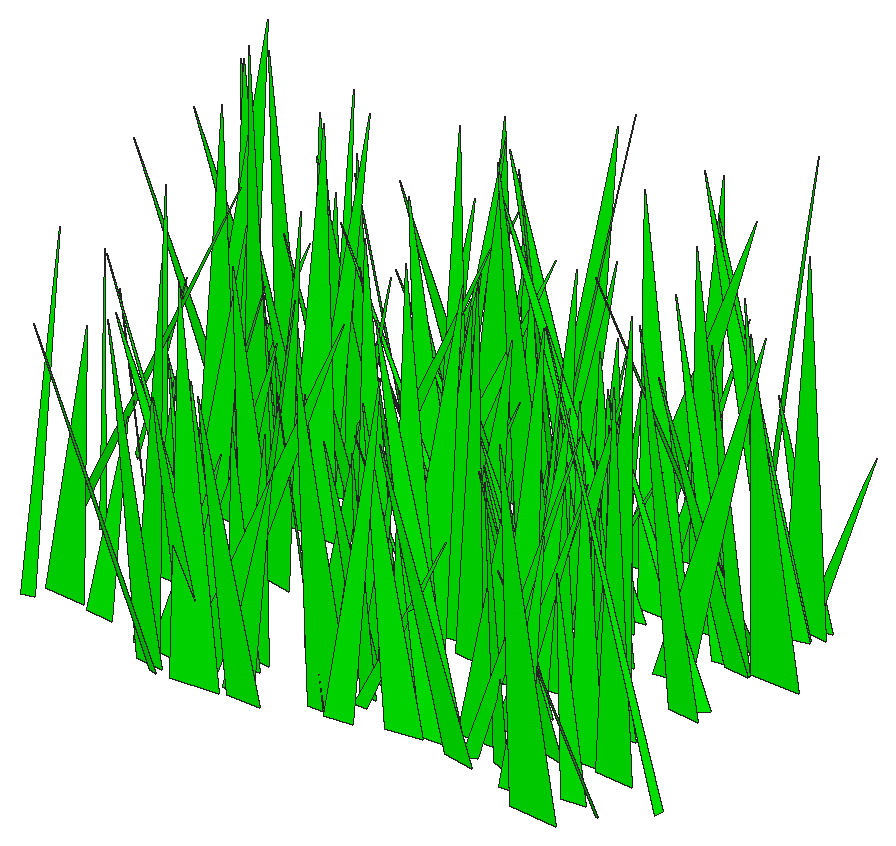
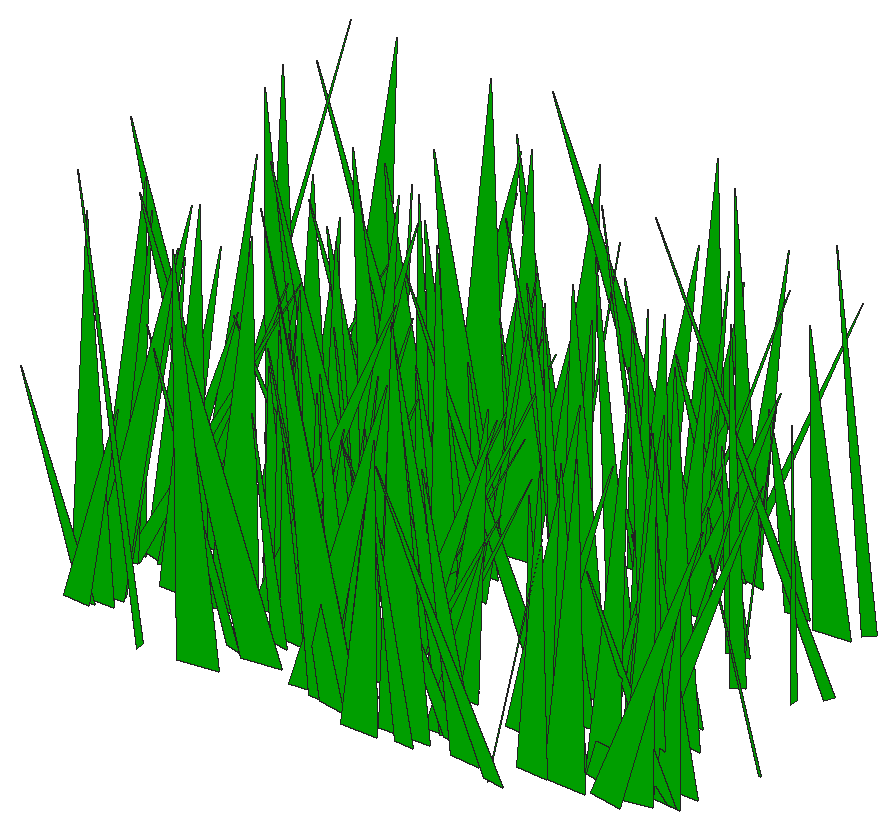
# SketchUp Ruby script. Lengths in inches.
U = 1.inch
M = Sketchup.active_model
def pt(a) = Geom::Point3d.new(a.map { |v| v * U })
def face(e, loops, mat)
  f = e.add_face(loops[0].map { |a| pt(a) })
  loops[1..].each { |l| e.add_face(l.map { |a| pt(a) }).erase! }
  f.material = f.back_material = mat if mat
  f
end
# faces: each face lists its corners as indices into pts; further lists are holes
def faces(e, pts, list, mat = nil) = list.each { |f| face(e, (f[0].is_a?(Array) ? f : [f]).map { |l| l.map { |i| pts[i] } }, mat) }
# xy, xz, yz: faces in a plane at the given z, y or x. An outline is a flat list of corners, or four numbers for a rectangle; further outlines are holes
def ring(l) = l.size == 4 ? [[l[0], l[1]], [l[2], l[1]], [l[2], l[3]], [l[0], l[3]]] : l.each_slice(2).to_a
def flat(e, list, mat, &to3) = list.each { |f| face(e, (f[0].is_a?(Array) ? f : [f]).map { |l| ring(l).map { |u, v| to3.(u, v) } }, mat) }
def xy(e, z, list, mat = nil) = flat(e, list, mat) { |x, y| [x, y, z] }
def xz(e, y, list, mat = nil) = flat(e, list, mat) { |x, z| [x, y, z] }
def yz(e, x, list, mat = nil) = flat(e, list, mat) { |y, z| [x, y, z] }
def lines(e, pts, list) = list.each { |a, b| e.add_line(pt(pts[a]), pt(pts[b])) }
# prism: a flat outline (further loops are holes) pulled along v
def prism(e, loops, v, mat = nil)
  f = face(e, loops, mat); d = Geom::Vector3d.new(v.map { |x| x * U })
  f.pushpull(f.normal.samedirection?(d) ? d.length : -d.length)
end
def box(e, o, s, mat = nil) = prism(e, [[o, [o[0] + s[0], o[1], o[2]], [o[0] + s[0], o[1] + s[1], o[2]], [o[0], o[1] + s[1], o[2]]]], [0, 0, s[2]], mat)
def at(x, y, z, deg = 0) = Geom::Transformation.translation(pt([x, y, z])) * Geom::Transformation.rotation(ORIGIN, Z_AXIS, deg.degrees)
def axes(o, x, y, z) = Geom::Transformation.new([*x, 0, *y, 0, *z, 0, *pt(o).to_a, 1])
def part(name) = M.definitions.add(name)
# library, detail: a bought-in or finely detailed component or shape, given as its bounding box
def library(name, o, s) = part(name).tap { |d| box(d.entities, o, s) }
def detail(e, o, s) = box(e.add_group.entities, o, s)
def put(e, d, t, mat = nil) = e.add_instance(d, t).tap { |i| i.material = mat if mat }
def group(e, t, mat = nil) = e.add_group.tap { |g| g.transformation = t; g.material = mat if mat }.entities
root = M.entities
M.materials.add("[0065_Lime]").color = [0, 255, 0]
c1 = part("fur_instance\#9")
p = [[0.8125,0,1.79],[0.67,-0.02,1.48],[0,-0.11,0],[0,0.11,0]]
faces(c1.entities,p,[[0,1,2,3]])
put(root,c1,axes([86.03,28.1875,1.48],[4.04083,0.10334,0.71067],[-0.84468,0.57426,0.37961],[-0.76857,-0.0878,3.31922]),"[0065_Lime]")
put(root,c1,axes([88.59,32.07,1.48],[-3.94525,-0.72329,0.33492],[5.16377,-0.55267,0.25148],[0.00431,0.07235,5.26929]),"[0065_Lime]")
put(root,c1,axes([87.08,31.14,1.48],[0.89992,-0.6126,0.18107],[4.3401,0.12899,0.35137],[-0.46837,0.0182,3.60385]),"[0065_Lime]")
put(root,c1,axes([87.77,31.65,1.48],[-5.27126,0.64585,1.86007],[-4.76084,-0.78731,0.23364],[1.92071,-0.17899,5.68396]),"[0065_Lime]")
put(root,c1,axes([89.39,29.05,1.48],[-5.37329,-0.53147,0.49477],[3.82303,-0.75334,0.35434],[0.24449,0.09936,5.33315]),"[0065_Lime]")
put(root,c1,axes([88.04,30.97,1.48],[0.57285,1.047,1.52629],[-7.66011,0.0985,-0.36204],[-0.60113,-0.25748,6.06786]),"[0065_Lime]")
put(root,c1,axes([87.96,24.23,1.48],[-5.20678,0.05391,1.90036],[-0.24332,-0.80109,0.32044],[2.35503,0.03643,4.23464]),"[0065_Lime]")
put(root,c1,axes([87.5,30.42,1.48],[1.19423,1.25105,0.91528],[-8.97397,0.16665,0.11422],[-0.00931,-0.15934,7.30591]),"[0065_Lime]")
put(root,c1,axes([87.07,31.14,1.48],[3.31324,0.45192,0.12553],[-3.21982,0.46497,0.13723],[0.00691,-0.03211,3.7534]),"[0065_Lime]")
put(root,c1,axes([89.58,31.27,1.48],[-2.8313,-0.4498,0.75727],[3.31009,-0.39968,0.23348],[0.39536,0.12512,3.46825]),"[0065_Lime]")
put(root,c1,axes([89.35,31.25,1.48],[4.48601,0.7755,2.98863],[-6.12778,0.72297,-0.20054],[-2.53145,-0.37579,5.78163]),"[0065_Lime]")
put(root,c1,axes([89.05,28.11,1.48],[-2.78497,-0.8522,3.3684],[7.24104,-0.42235,0.38055],[1.2235,0.55979,5.41505]),"[0065_Lime]")
put(root,c1,axes([88.17,28.92,1.48],[4.25422,-0.04589,0.62894],[0.27567,0.60656,0.24919],[-0.79279,-0.03533,3.46166]),"[0065_Lime]")
put(root,c1,axes([88.69,19.89,1.48],[7.16155,-0.18947,2.24815],[1.59238,1.07053,-0.33303],[-2.63082,0.13221,5.91829]),"[0065_Lime]")
put(root,c1,axes([89.9,28.91,1.48],[-6.41024,-0.72474,2.92404],[5.66582,-0.9786,0.09049],[2.7244,0.32992,6.69179]),"[0065_Lime]")
put(root,c1,axes([90.01,32.15,1.48],[1.06489,-0.86721,2.0596],[6.63418,0.17535,0.20448],[-0.69739,0.34385,5.09006]),"[0065_Lime]")
put(root,c1,axes([89.72,24.6,1.48],[-6.42583,0.25596,2.56922],[-1.98471,-0.99997,0.05395],[3.05869,-0.11112,5.43254]),"[0065_Lime]")
put(root,c1,axes([90.54,23.32,1.48],[-5.24025,-0.12439,1.38818],[0.80005,-0.77419,-0.32639],[1.74817,-0.01856,4.31054]),"[0065_Lime]")
put(root,c1,axes([89.62,27.03,1.48],[2.51456,0.77635,0.8023],[-5.5838,0.36135,-0.13764],[-0.56446,-0.11612,4.93568]),"[0065_Lime]")
put(root,c1,axes([89.54,20.53,1.48],[0.63715,-0.86567,0.6252],[6.19645,0.08196,-0.37544],[0.38378,0.11385,5.0238]),"[0065_Lime]")
put(root,c1,axes([91.32,25.14,1.48],[-4.16997,0.13533,0.69258],[-1.02836,-0.59488,-0.20161],[0.77135,-0.06148,3.47535]),"[0065_Lime]")
put(root,c1,axes([87.27,23.48,1.48],[9.017,-0.09495,0.44591],[0.68586,1.26911,-0.12098],[-0.53545,0.02663,7.35411]),"[0065_Lime]")
put(root,c1,axes([91.93,33.24,1.48],[-5.20309,-0.09303,1.05154],[0.59415,-0.75284,-0.28659],[1.32532,-0.02771,4.25674]),"[0065_Lime]")
put(root,c1,axes([90.71,31.09,1.48],[2.09408,-0.8014,0.72809],[5.74409,0.30262,0.23064],[-0.57723,0.10406,4.93651]),"[0065_Lime]")
put(root,c1,axes([91.21,32.15,1.48],[-3.10372,-0.68812,1.8346],[5.2342,-0.47225,-0.07664],[1.29263,0.26005,4.71534]),"[0065_Lime]")
put(root,c1,axes([90.89,23.12,1.48],[-1.58701,0.49138,1.36255],[-3.73837,-0.26141,0.27803],[1.02908,-0.19183,3.11127]),"[0065_Lime]")
put(root,c1,axes([91.02,20.25,1.48],[0.34432,0.60128,0.49992],[-4.31408,0.04225,0.2632],[0.27666,-0.08952,3.48194]),"[0065_Lime]")
put(root,c1,axes([90.48,26.84,1.48],[2.13067,-0.53653,0.37097],[3.84241,0.29416,-0.34537],[0.1516,0.08493,3.53984]),"[0065_Lime]")
put(root,c1,axes([92.04,26.2,1.48],[0.50197,-0.76027,1.37562],[5.63187,0.09401,0.38125],[-0.64443,0.22937,4.40337]),"[0065_Lime]")
put(root,c1,axes([93.5625,22.1,1.48],[-4.52451,0.50099,0.28299],[-3.58217,-0.63323,-0.32904],[0.02176,-0.07491,4.67404]),"[0065_Lime]")
put(root,c1,axes([92.68,30.49,1.48],[-0.96712,-1.02503,0.3105],[7.29873,-0.13343,0.28177],[-0.29375,0.05952,5.97885]),"[0065_Lime]")
put(root,c1,axes([94.25,18.65,1.48],[-6.30246,-0.24518,0.48424],[1.78851,-0.88542,0.37897],[0.44746,0.08562,5.30583]),"[0065_Lime]")
put(root,c1,axes([93.55,28.98,1.48],[-4.67422,-0.41949,0.77765],[3.07015,-0.66133,0.25562],[0.63279,0.10996,4.50412]),"[0065_Lime]")
put(root,c1,axes([91.95,29.78,1.48],[7.64496,-0.26622,2.61897],[2.13429,1.15701,-0.18107],[-3.0661,0.14159,6.40407]),"[0065_Lime]")
put(root,c1,axes([94.74,21.09,1.48],[-7.30199,0.04274,0.76879],[-0.26383,-1.0338,0.26771],[0.95717,0.04107,5.93865]),"[0065_Lime]")
put(root,c1,axes([92.59,30.31,1.48],[-2.98365,-0.45574,1.59582],[3.49222,-0.46692,-0.14825],[1.47394,0.18373,3.58161]),"[0065_Lime]")
put(root,c1,axes([91.89,29.12,1.48],[7.25302,-0.57073,1.92647],[4.19021,1.06216,0.10651],[-2.1327,0.14589,6.76094]),"[0065_Lime]")
put(root,c1,axes([92.83,27.71,1.48],[-2.87939,1.03833,2.40511],[-7.82216,-0.45076,0.32479],[1.46925,-0.3649,6.4426]),"[0065_Lime]")
put(root,c1,axes([93.88,18.95,1.48],[-4.81384,-0.61573,1.676],[4.63408,-0.70422,0.13728],[1.40405,0.21323,5.29314]),"[0065_Lime]")
put(root,c1,axes([93.29,19.57,1.48],[5.72947,0.66066,2.42178],[-5.06339,0.86801,-0.00891],[-2.30906,-0.26411,6.0287]),"[0065_Lime]")
put(root,c1,axes([94.0625,21.62,1.48],[-2.35642,0.53998,1.63788],[-4.29031,-0.33785,-0.35163],[0.64414,-0.27487,3.64976]),"[0065_Lime]")
put(root,c1,axes([94.35,21.02,1.48],[-2.68065,0.46037,0.38934],[-3.27201,-0.38158,0.21344],[0.5069,-0.02846,3.4367]),"[0065_Lime]")
put(root,c1,axes([91.73,33.25,1.48],[4.99894,0.51633,0.09697],[-3.67616,0.70236,0.07104],[-0.04431,-0.01981,5.04603]),"[0065_Lime]")
put(root,c1,axes([94.77,31.97,1.48],[-2.33051,0.57135,0.33218],[-4.08624,-0.32507,-0.23277],[-0.04652,-0.06976,3.80501]),"[0065_Lime]")
put(root,c1,axes([93.15,32.78,1.48],[2.93751,0.70108,0.9852],[-5.09923,0.42123,0.01537],[-0.59788,-0.14804,4.70946]),"[0065_Lime]")
put(root,c1,axes([93.83,24.81,1.48],[-5.24364,-0.63249,2.99099],[5.05891,-0.83929,-0.07906],[2.86155,0.32477,5.62059]),"[0065_Lime]")
put(root,c1,axes([95.17,19.42,1.48],[-5.76861,0.18281,1.60389],[-1.23906,-0.85663,0.32311],[2.01126,-0.00342,4.79925]),"[0065_Lime]")
put(root,c1,axes([93.83,19.65,1.48],[2.04566,0.60081,0.00556],[-4.27557,0.28744,0.02824],[0.02837,-0.00297,3.85534]),"[0065_Lime]")
put(root,c1,axes([95.64,29.99,1.48],[-1.88741,0.91938,0.41555],[-6.56263,-0.26403,-0.14749],[-0.03316,-0.07603,5.53705]),"[0065_Lime]")
put(root,c1,axes([95.7,18.93,1.48],[-2.98711,-0.68925,0.80252],[4.96925,-0.42751,-0.06573],[0.58313,0.1124,4.67103]),"[0065_Lime]")
put(root,c1,axes([96.9,31.13,1.48],[-4.86899,0.11572,0.16903],[-0.83851,-0.68199,-0.33524],[0.13538,-0.06201,4.00274]),"[0065_Lime]")
put(root,c1,axes([96.79,31.51,1.48],[-4.52046,-0.72566,0.40008],[5.18576,-0.63453,0.20271],[0.13575,0.07509,5.57892]),"[0065_Lime]")
put(root,c1,axes([94.98,31.66,1.48],[3.7016,0.2066,1.14464],[-1.42051,0.55619,-0.3245],[-1.45743,-0.01737,3.22346]),"[0065_Lime]")
put(root,c1,axes([95.69,18.76,1.48],[1.77449,-0.98089,3.05276],[7.83983,0.29649,0.17716],[-1.16223,0.50238,5.856]),"[0065_Lime]")
put(root,c1,axes([94.32,31.9,1.48],[6.98938,-0.44614,1.69614],[3.31092,1.01631,-0.06941],[-1.86182,0.13249,6.24395]),"[0065_Lime]")
put(root,c1,axes([97.31,28.75,1.48],[-4.58533,-0.17957,0.22713],[1.28519,-0.64509,0.07713],[0.24342,0.02339,3.87113]),"[0065_Lime]")
put(root,c1,axes([95.11,33.125,1.48],[3.44674,0.43758,1.26928],[-3.35812,0.49936,0.26484],[-0.92475,-0.18245,3.76911]),"[0065_Lime]")
put(root,c1,axes([95.38,32.76,1.48],[0.6225,-1.16517,1.07209],[8.3925,0.08091,-0.27771],[0.24611,0.18817,6.75811]),"[0065_Lime]")
put(root,c1,axes([94.14,32.09,1.48],[4.70239,0.5043,0.09383],[-3.59067,0.66055,0.09974],[-0.01727,-0.02353,4.81066]),"[0065_Lime]")
put(root,c1,axes([96.13,20.46,1.48],[0.86751,-0.7228,0.53652],[5.16693,0.12851,0.27388],[-0.44412,0.08327,4.23433]),"[0065_Lime]")
put(root,c1,axes([95.29,21.59,1.48],[-6.1048,-0.27843,3.1373],[2.11287,-1.0083,-0.27832],[3.78658,0.11373,5.21332]),"[0065_Lime]")
put(root,c1,axes([96.64,33.28,1.48],[-1.92502,0.75297,1.78022],[-5.76376,-0.27916,-0.16715],[0.53227,-0.2997,4.62844]),"[0065_Lime]")
put(root,c1,axes([96.07,21.03,1.48],[-0.49663,-0.67233,0.88373],[4.87395,-0.08523,-0.3605],[0.56361,0.14461,3.89615]),"[0065_Lime]")
put(root,c1,axes([99.14,27.45,1.48],[-7.16847,0.07697,0.30495],[-0.54164,-1.00857,0.10615],[0.3837,0.0143,5.84696]),"[0065_Lime]")
put(root,c1,axes([93.95,28.14,1.48],[7.45779,-0.35097,0.2333],[2.48234,1.04795,0.32467],[-0.39846,-0.04044,6.38919]),"[0065_Lime]")
put(root,c1,axes([97.35,18.92,1.48],[-2.46713,-0.78531,0.91792],[5.69029,-0.34997,0.0861],[0.3572,0.15115,4.96842]),"[0065_Lime]")
put(root,c1,axes([96.51,29.41,1.48],[6.69522,-0.63939,2.8413],[4.98924,1.02135,-0.07697],[-2.83087,0.28786,6.58422]),"[0065_Lime]")
put(root,c1,axes([95.8,29.52,1.48],[4.45032,-0.60961,0.8059],[4.36425,0.63637,0.18455],[-0.86934,0.074,5.05199]),"[0065_Lime]")
put(root,c1,axes([97.29,22.42,1.48],[-2.1606,-0.65244,1.23513],[4.81878,-0.32297,-0.13947],[0.8024,0.18274,4.16334]),"[0065_Lime]")
put(root,c1,axes([98.05,32.4375,1.48],[-6.44509,-0.25277,1.83432],[1.95631,-0.95304,0.14724],[2.11994,0.11101,5.44089]),"[0065_Lime]")
put(root,c1,axes([97.23,28.5625,1.48],[3.46289,0.39438,1.48863],[-3.01998,0.52757,-0.03533],[-1.45127,-0.15679,3.62557]),"[0065_Lime]")
put(root,c1,axes([99.34,27.22,1.48],[-4.93591,-0.10561,0.07686],[0.75703,-0.69088,0.35484],[0.02738,0.0626,4.04568]),"[0065_Lime]")
put(root,c1,axes([96.52,23.78,1.48],[6.35659,0.55025,1.45954],[-3.94858,0.92398,-0.29436],[-1.72114,-0.08756,6.06575]),"[0065_Lime]")
put(root,c1,axes([99.25,32.31,1.48],[-4.77874,0.84226,0.2925],[-5.99757,-0.67265,0.0721],[0.29354,-0.03173,6.23502]),"[0065_Lime]")
put(root,c1,axes([98.61,25.18,1.48],[-6.59327,-0.28209,1.56863],[1.99347,-0.96474,-0.26958],[1.94294,0.03258,5.59965]),"[0065_Lime]")
put(root,c1,axes([96.93,19.1875,1.48],[1.56737,-0.67288,0.6223],[4.84771,0.2145,-0.30665],[0.12507,0.11855,4.08696]),"[0065_Lime]")
put(root,c1,axes([95.14,19.74,1.48],[7.49911,-0.68292,0.41068],[4.87795,1.05389,-0.20878],[-0.2837,0.06888,7.26587]),"[0065_Lime]")
put(root,c1,axes([98.33,30.73,1.48],[-0.36242,0.81621,0.08718],[-5.80927,-0.05076,-0.05253],[-0.05779,-0.01559,4.73366]),"[0065_Lime]")
put(root,c1,axes([98.79,27.62,1.48],[-3.13529,-0.49774,1.52243],[3.83228,-0.46996,0.07325],[1.16778,0.20592,3.8471]),"[0065_Lime]")
put(root,c1,axes([99.44,19.91,1.48],[-5.81231,-0.14491,1.45485],[1.20351,-0.8479,0.35128],[1.67752,0.10622,4.78878]),"[0065_Lime]")
put(root,c1,axes([98.07,32.6,1.48],[2.15064,1.21441,0.14312],[-8.6398,0.3028,-0.19535],[-0.27558,-0.01583,7.2416]),"[0065_Lime]")
put(root,c1,axes([99.375,22.21,1.48],[-2.55361,-0.60704,0.26531],[4.31243,-0.36126,-0.23464],[0.41455,0.01872,4.07521]),"[0065_Lime]")
put(root,c1,axes([98.09,32.7,1.48],[3.66492,0.61612,0.90487],[-4.46208,0.52544,-0.03086],[-0.74307,-0.11645,4.64821]),"[0065_Lime]")
put(root,c1,axes([99.3125,22.64,1.48],[-4.21624,1.01487,2.01393],[-7.48842,-0.62718,0.21788],[1.48885,-0.28051,6.79908]),"[0065_Lime]")
put(root,c1,axes([97.49,27.8,1.48],[4.4356,-0.266,0.15227],[1.88004,0.62319,0.24381],[-0.28958,-0.02846,3.91522]),"[0065_Lime]")
put(root,c1,axes([98.73,31.34,1.48],[4.06229,-0.59453,1.3386],[4.35948,0.59745,0.13825],[-1.2666,0.14956,4.76902]),"[0065_Lime]")
put(root,c1,axes([99.77,19.88,1.48],[-0.48716,-1.05909,0.61167],[7.57237,-0.06561,0.18373],[-0.17803,0.10746,6.14078]),"[0065_Lime]")
put(root,c1,axes([99.07,22.46,1.48],[3.60187,0.40609,1.09838],[-2.98977,0.52954,-0.07358],[-1.112,-0.10839,3.75557]),"[0065_Lime]")
put(root,c1,axes([97.88,31.875,1.48],[9.08789,0.18976,1.8378],[-1.3943,1.31498,0.01214],[-2.23256,-0.0488,7.47337]),"[0065_Lime]")
put(root,c1,axes([99.96,21.33,1.48],[-3.57418,-0.39045,1.45708],[3.0397,-0.53388,0.13951],[1.3,0.17484,3.67986]),"[0065_Lime]")
put(root,c1,axes([99.39,23.96,1.48],[2.52048,-0.47153,0.541],[3.36444,0.36269,0.22159],[-0.61914,0.05129,3.40654]),"[0065_Lime]")
put(root,c1,axes([100.52,28.47,1.48],[-4.96564,-1.01095,1.93745],[7.41374,-0.73099,-0.20922],[1.57182,0.25406,7.10758]),"[0065_Lime]")
put(root,c1,axes([101.8,22.69,1.48],[-4.96831,0.00753,0.31786],[-0.07995,-0.69866,-0.2724],[0.38624,-0.04779,4.03233]),"[0065_Lime]")
put(root,c1,axes([99.48,25.42,1.48],[3.80749,-0.88549,1.00747],[6.35385,0.54883,0.27603],[-0.93437,0.1238,5.98245]),"[0065_Lime]")
put(root,c1,axes([99.4,26.99,1.48],[1.5064,-0.91139,0.26779],[6.4863,0.20879,-0.33085],[0.32234,0.05792,5.40607]),"[0065_Lime]")
put(root,c1,axes([103.09,29.5,1.48],[-7.20756,0.53099,0.20381],[-3.76765,-1.01304,0.283],[0.38334,0.02699,6.61356]),"[0065_Lime]")
put(root,c1,axes([101.37,29.86,1.48],[-4.19113,0.24642,0.83769],[-1.75907,-0.60561,0.14656],[1.0206,-0.03187,3.69261]),"[0065_Lime]")
put(root,c1,axes([100.18,19.74,1.48],[-5.21221,0.52408,3.00978],[-4.14292,-0.8604,0.27331],[3.23078,-0.25781,5.20614]),"[0065_Lime]")
put(root,c1,axes([100.86,24.87,1.48],[5.2899,0.68458,2.31174],[-5.15837,0.80864,-0.21424],[-2.28098,-0.24109,5.84573]),"[0065_Lime]")
put(root,c1,axes([100.49,22.94,1.48],[0.74059,1.18616,0.87624],[-8.50522,0.09817,0.30313],[0.28017,-0.15526,6.88603]),"[0065_Lime]")
put(root,c1,axes([102.14,20.27,1.48],[-2.00366,0.86038,0.7845],[-6.197,-0.275,-0.36601],[-0.1332,-0.14837,5.22757]),"[0065_Lime]")
put(root,c1,axes([101.32,30.49,1.48],[0.96996,0.53402,0.84598],[-3.9249,0.14416,-0.07176],[-0.34557,-0.1384,3.18954]),"[0065_Lime]")
put(root,c1,axes([103.04,26.02,1.48],[-3.3694,0.40735,0.10034],[-2.8989,-0.47147,-0.27056],[-0.12377,-0.04672,3.60535]),"[0065_Lime]")
put(root,c1,axes([101.13,27.57,1.48],[5.20611,-0.04577,1.54913],[0.49937,0.77488,-0.3432],[-1.86649,0.07965,4.22909]),"[0065_Lime]")
put(root,c1,axes([102.22,20.83,1.48],[-2.02806,1.27509,1.24963],[-9.19603,-0.28959,0.02683],[0.36771,-0.20965,7.56316]),"[0065_Lime]")
put(root,c1,axes([100.14,20.78,1.48],[4.05172,-0.24086,0.16976],[1.72615,0.56698,-0.3023],[-0.04656,0.05954,3.56573]),"[0065_Lime]")
put(root,c1,axes([100.8125,29.6,1.48],[5.18578,0.26596,1.00114],[-1.8663,0.7488,-0.2696],[-1.27054,-0.01437,4.48226]),"[0065_Lime]")
put(root,c1,axes([101.75,28.8,1.48],[3.18601,-0.39642,1.19727],[2.86771,0.48455,0.32695],[-1.37901,0.09176,3.44603]),"[0065_Lime]")
put(root,c1,axes([103.38,20.52,1.48],[-4.95266,0.95785,0.21261],[-6.80269,-0.69687,0.35626],[0.50794,0.00652,6.84444]),"[0065_Lime]")
put(root,c1,axes([101.48,30.84,1.48],[3.52892,0.37904,1.08038],[-2.80358,0.5188,-0.0402],[-1.08648,-0.10758,3.6128]),"[0065_Lime]")
put(root,c1,axes([102.6,28.85,1.48],[-2.41907,0.6927,0.73234],[-4.94324,-0.35291,0.3821],[0.82251,-0.08369,4.45025]),"[0065_Lime]")
put(root,c1,axes([102.21,29.37,1.48],[1.06039,-0.73807,1.72179],[5.65967,0.14852,-0.1728],[-0.19466,0.29768,4.35525]),"[0065_Lime]")
put(root,c1,axes([103.68,30.2,1.48],[-2.9082,1.16047,0.54886],[-8.26636,-0.41325,0.2984],[0.57097,-0.07218,7.11569]),"[0065_Lime]")
put(root,c1,axes([104.33,20.02,1.48],[-4.09177,-0.69665,0.43226],[4.96433,-0.57822,-0.13422],[0.46585,0.04276,5.22706]),"[0065_Lime]")
put(root,c1,axes([102.58,33.2,1.48],[-4.66468,0.77037,3.33815],[-6.29486,-0.75711,0.0348],[2.69687,-0.43471,5.8551]),"[0065_Lime]")
put(root,c1,axes([103.1,28.89,1.48],[0.69667,-0.66825,0.38461],[4.77875,0.0966,-0.10332],[0.05777,0.06832,3.90823]),"[0065_Lime]")
put(root,c1,axes([104.68,23.57,1.48],[-4.3671,0.26341,0.49924],[-1.86795,-0.61959,0.14336],[0.6337,-0.01105,3.86304]),"[0065_Lime]")
put(root,c1,axes([102.89,24.41,1.48],[4.91815,-0.81935,1.56316],[5.95783,0.72048,0.25207],[-1.48228,0.17729,6.19968]),"[0065_Lime]")
put(root,c1,axes([103.84,27.6,1.48],[-2.00216,0.70326,0.6112],[-5.01797,-0.29061,0.3289],[0.65736,-0.07645,4.37225]),"[0065_Lime]")
put(root,c1,axes([101.23,31.97,1.48],[6.65886,-0.86181,0.24522],[6.13603,0.93626,0.01488],[-0.23414,0.02681,7.36374]),"[0065_Lime]")
put(root,c1,axes([102.41,31.8,1.48],[5.56727,0.36952,0.80735],[-2.68225,0.79094,0.10733],[-0.84018,-0.07654,5.0071]),"[0065_Lime]")
put(root,c1,axes([104.38,27.32,1.48],[0.16459,0.62466,1.43978],[-4.77431,0.03793,-0.19034],[-0.31708,-0.2469,3.6134]),"[0065_Lime]")
put(root,c1,axes([104.1,24.88,1.48],[2.24832,-0.76043,1.10874],[5.51859,0.33367,0.26428],[-0.8302,0.15862,4.75937]),"[0065_Lime]")
put(root,c1,axes([103.72,23.92,1.48],[0.54033,0.90156,0.50765],[-6.43563,0.07039,0.34344],[0.37045,-0.0922,5.22606]),"[0065_Lime]")
put(root,c1,axes([102.41,26.8,1.48],[4.76991,-0.2041,0.01041],[1.44943,0.66838,-0.30059],[0.09544,0.0502,4.04466]),"[0065_Lime]")
put(root,c1,axes([104.04,21.28,1.48],[2.06177,-0.89065,0.07791],[6.33876,0.28954,-0.07654],[0.05987,0.01689,5.42104]),"[0065_Lime]")
put(root,c1,axes([107.94,29.4,1.48],[-7.08772,-0.3527,0.04583],[2.50863,-0.99395,0.37463],[-0.10074,0.06364,6.1046]),"[0065_Lime]")
put(root,c1,axes([103.3125,25.06,1.48],[6.10677,-0.59177,0.5403],[4.18497,0.86317,0.38286],[-0.814,-0.00178,6.02181]),"[0065_Lime]")
put(root,c1,axes([106.29,21.86,1.48],[-4.17134,-0.57999,0.3271],[4.10233,-0.58883,-0.37218],[0.60756,-0.00619,4.7588]),"[0065_Lime]")
put(root,c1,axes([105.5,20.48,1.48],[4.49285,0.33175,2.30532],[-2.88791,0.70681,0.31556],[-2.2948,-0.23998,4.11631]),"[0065_Lime]")
put(root,c1,axes([105.42,30.27,1.48],[1.77733,-1.05744,1.88494],[7.81336,0.2782,0.3552],[-0.97546,0.30168,6.27955]),"[0065_Lime]")
put(root,c1,axes([105.39,25.34,1.48],[-2.97309,-0.49592,1.41951],[3.73665,-0.45223,-0.116],[1.2404,0.17365,3.75182]),"[0065_Lime]")
put(root,c1,axes([107.28,31.5,1.48],[-6.95931,0.76227,1.42207],[-5.55597,-0.99379,-0.13954],[1.27108,-0.17038,7.17606]),"[0065_Lime]")
put(root,c1,axes([104.23,22.28,1.48],[4.48765,0.50862,0.7105],[-3.69807,0.63125,0.31208],[-0.43476,-0.11933,4.67932]),"[0065_Lime]")
put(root,c1,axes([104.58,33.34,1.48],[8.91937,0.01062,2.2683],[-0.04937,1.31311,-0.0776],[-2.78921,0.01072,7.25498]),"[0065_Lime]")
put(root,c1,axes([107.21,31.67,1.48],[-5.65899,0.79229,1.14548],[-5.73978,-0.80524,-0.09856],[0.91064,-0.1519,6.49716]),"[0065_Lime]")
put(root,c1,axes([106.76,29.17,1.48],[-5.87453,0.53253,1.3759],[-3.85158,-0.85299,0.18209],[1.54554,-0.10159,5.68355]),"[0065_Lime]")
put(root,c1,axes([107.29,29.04,1.48],[-3.9052,-0.59326,0.61456],[4.27679,-0.54947,0.20729],[0.32384,0.10239,4.67346]),"[0065_Lime]")
put(root,c1,axes([108,26.64,1.48],[-5.58296,0.25364,0.5668],[-1.85117,-0.7872,-0.26],[0.56302,-0.07311,4.76563]),"[0065_Lime]")
put(root,c1,axes([104.45,20.39,1.48],[7.499,-0.26761,0.90701],[1.9202,1.06476,0.02287],[-1.08774,0.0347,6.29338]),"[0065_Lime]")
put(root,c1,axes([107.26,23.98,1.48],[-3.21405,0.4147,0.93476],[-3.04779,-0.46755,0.01692],[0.861,-0.10699,3.54926]),"[0065_Lime]")
put(root,c1,axes([106.51,24.23,1.48],[3.94363,1.00567,2.04061],[-7.43718,0.5906,-0.24353],[-1.48421,-0.2873,6.64233]),"[0065_Lime]")
put(root,c1,axes([107.67,32.39,1.48],[-2.14254,0.56336,0.45677],[-4.04828,-0.298,-0.24824],[-0.00713,-0.0898,3.68922]),"[0065_Lime]")
put(root,c1,axes([107.35,29.11,1.48],[-4.93288,-0.48512,1.89554],[3.82543,-0.72845,0.33973],[1.64783,0.23886,4.88573]),"[0065_Lime]")
put(root,c1,axes([107.67,26.125,1.48],[-5.27761,-0.72009,1.9518],[5.43563,-0.77329,0.16486],[1.57233,0.25629,5.98137]),"[0065_Lime]")
put(root,c1,axes([107.31,22.14,1.48],[0.44921,0.80059,1.6936],[-6.05805,0.07418,-0.11192],[-0.3096,-0.28996,4.6474]),"[0065_Lime]")
put(root,c1,axes([106.68,19.63,1.48],[3.04367,-0.62246,1.27052],[4.64449,0.43787,-0.17322],[-0.70107,0.1984,4.36839]),"[0065_Lime]")
put(root,c1,axes([107.96,29.71,1.48],[-6.43081,0.36161,2.141],[-2.7927,-0.9643,-0.09243],[2.39822,-0.15325,5.63344]),"[0065_Lime]")
put(root,c1,axes([107.32,32.1,1.48],[-2.25967,-0.99592,2.08586],[7.43324,-0.35672,-0.37932],[1.24736,0.32158,6.03911]),"[0065_Lime]")
put(root,c1,axes([109.44,19.95,1.48],[-4.55458,-0.11085,0.0904],[0.79548,-0.63771,0.31472],[0.04307,0.05624,3.74672]),"[0065_Lime]")
put(root,c1,axes([107.99,18.85,1.48],[-1.59816,-1.11305,0.64061],[7.95105,-0.22861,-0.1859],[0.38079,0.10206,6.57033]),"[0065_Lime]")
put(root,c1,axes([106.09,27.58,1.48],[6.1316,-0.79879,0.65706],[5.70617,0.8662,0.05412],[-0.6378,0.07028,6.80097]),"[0065_Lime]")
put(root,c1,axes([108.42,20.18,1.48],[-2.24557,0.52252,1.08503],[-3.90331,-0.32671,-0.07286],[0.6092,-0.16722,3.5327]),"[0065_Lime]")
put(root,c1,axes([108.47,21.95,1.48],[4.11298,0.86601,2.44704],[-6.58356,0.63664,-0.22834],[-1.92076,-0.32773,6.02256]),"[0065_Lime]")
put(root,c1,axes([108.58,29.16,1.48],[-0.29511,-1.12407,0.14712],[8.00143,-0.04159,-0.02921],[0.04257,0.02521,6.51125]),"[0065_Lime]")
put(root,c1,axes([110.6875,21.23,1.48],[-9.10938,0.03837,1.49479],[-0.31316,-1.30541,-0.13977],[1.83127,-0.03236,7.4117]),"[0065_Lime]")
put(root,c1,axes([107.35,32.28,1.48],[4.11261,-0.26639,0.14691],[1.86991,0.57632,0.3834],[-0.36061,-0.04963,3.66355]),"[0065_Lime]")
